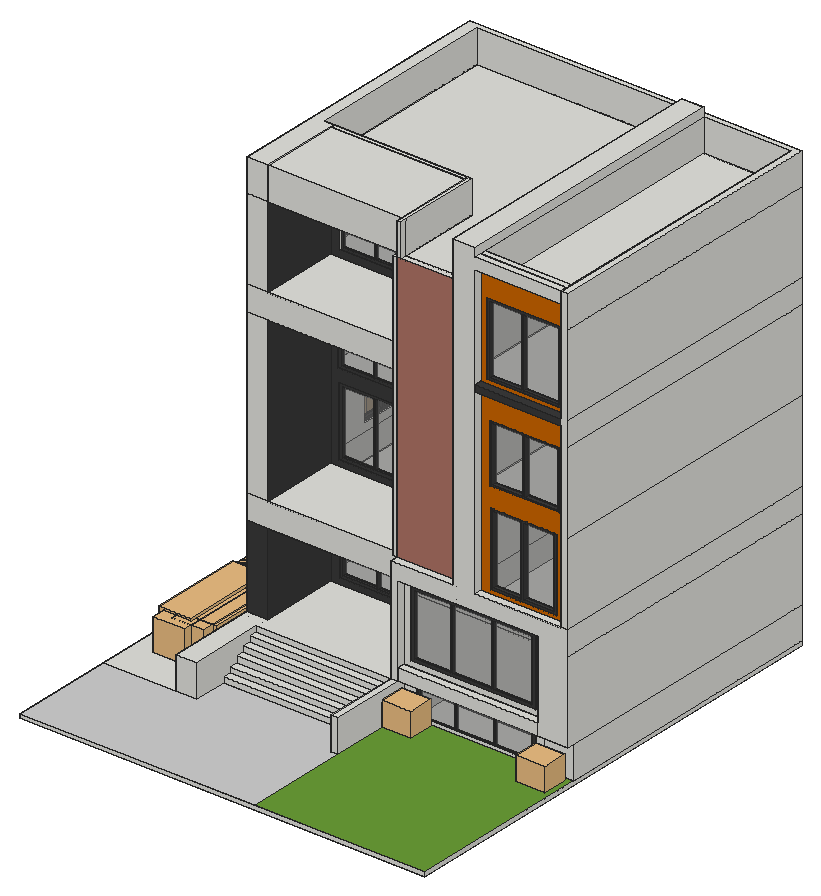
# SketchUp Ruby script. Lengths in inches.
U = 1.inch
M = Sketchup.active_model
def pt(a) = Geom::Point3d.new(a.map { |v| v * U })
def face(e, loops, mat)
  f = e.add_face(loops[0].map { |a| pt(a) })
  loops[1..].each { |l| e.add_face(l.map { |a| pt(a) }).erase! }
  f.material = f.back_material = mat if mat
  f
end
# faces: each face lists its corners as indices into pts; further lists are holes
def faces(e, pts, list, mat = nil) = list.each { |f| face(e, (f[0].is_a?(Array) ? f : [f]).map { |l| l.map { |i| pts[i] } }, mat) }
# xy, xz, yz: faces in a plane at the given z, y or x. An outline is a flat list of corners, or four numbers for a rectangle; further outlines are holes
def ring(l) = l.size == 4 ? [[l[0], l[1]], [l[2], l[1]], [l[2], l[3]], [l[0], l[3]]] : l.each_slice(2).to_a
def flat(e, list, mat, &to3) = list.each { |f| face(e, (f[0].is_a?(Array) ? f : [f]).map { |l| ring(l).map { |u, v| to3.(u, v) } }, mat) }
def xy(e, z, list, mat = nil) = flat(e, list, mat) { |x, y| [x, y, z] }
def xz(e, y, list, mat = nil) = flat(e, list, mat) { |x, z| [x, y, z] }
def yz(e, x, list, mat = nil) = flat(e, list, mat) { |y, z| [x, y, z] }
def lines(e, pts, list) = list.each { |a, b| e.add_line(pt(pts[a]), pt(pts[b])) }
# prism: a flat outline (further loops are holes) pulled along v
def prism(e, loops, v, mat = nil)
  f = face(e, loops, mat); d = Geom::Vector3d.new(v.map { |x| x * U })
  f.pushpull(f.normal.samedirection?(d) ? d.length : -d.length)
end
def box(e, o, s, mat = nil) = prism(e, [[o, [o[0] + s[0], o[1], o[2]], [o[0] + s[0], o[1] + s[1], o[2]], [o[0], o[1] + s[1], o[2]]]], [0, 0, s[2]], mat)
def at(x, y, z, deg = 0) = Geom::Transformation.translation(pt([x, y, z])) * Geom::Transformation.rotation(ORIGIN, Z_AXIS, deg.degrees)
def axes(o, x, y, z) = Geom::Transformation.new([*x, 0, *y, 0, *z, 0, *pt(o).to_a, 1])
def part(name) = M.definitions.add(name)
# library, detail: a bought-in or finely detailed component or shape, given as its bounding box
def library(name, o, s) = part(name).tap { |d| box(d.entities, o, s) }
def detail(e, o, s) = box(e.add_group.entities, o, s)
def put(e, d, t, mat = nil) = e.add_instance(d, t).tap { |i| i.material = mat if mat }
def group(e, t, mat = nil) = e.add_group.tap { |g| g.transformation = t; g.material = mat if mat }.entities
root = M.entities
M.materials.add("[Carrera Marble]").color = [207, 207, 207]
M.materials.add("[Color C06]").color = [204, 102, 0]
M.materials.add("[Color M07]").color = [58, 58, 58]
M.materials.add("[Grass Dark Green]").color = [106, 157, 55]
M.materials.add("[Groundcover Rock Crushed Multi]").color = [143, 133, 129]
M.materials.add("[Polished Concrete New]").color = [200, 200, 203]
M.materials.add("[Stone Flagstone Ashlar]").color = [175, 116, 102]
M.materials.add("[Translucent Glass Gray]").color = [128, 128, 128]
M.materials["[Translucent Glass Gray]"].alpha = 0.5
c1 = library("Vasos",[-24.5625,-15.95,-1.45],[31.57,37.11,26.14])
c2 = library("Leafy branch",[-35.17,-3.01,-3.57],[143.18,161.35,119.45])
c3 = library("Group\#55",[5.86,-0.04,-1.79],[34.39,19.68,504.85])
c4 = library("Group\#24",[28.02,-2.92,-0.02],[141.73,84.93,456.9])
c5 = library("Group\#66",[-11.6875,-1.03,-0.36],[108.82,105.43,84.06])
c6 = library("Group\#74",[28.02,-2.92,-0.02],[141.73,84.93,456.9])
c7 = library("Group\#19",[-11.6875,-1.03,-0.36],[108.82,105.43,84.06])
c8 = library("Group\#65",[-11.6875,-1.03,-0.36],[108.82,105.43,84.06])
c9 = part("BROADLEAF TREE 4")
g1 = group(c9.entities,at(835.71,714.57,-6.32))
put(g1,c2,at(175.35,181.4,81.93,-120))
put(g1,c2,at(98.01,135.17,98.79))
put(g1,c2,at(125.27,89.16,75.51,60))
put(g1,c3,axes([114.37,132.6,1.2],[1.053,0,0],[0,0.702,0],[0,0,0.67275]))
g2 = group(g1,at(131.4375,132.24,187.74))
detail(g2,[0.38,-62.11,4.18],[9.04,69.09,65.1])
g3 = group(g1,at(138.38,139.84,128.99))
detail(g3,[-52.45,-27.55,5.12],[58.39,28.31,68.09])
g4 = group(g1,at(143.59,136.18,156.43))
p = [[-4.06,0.97,6.8125],[-3.16,1.92,5.12],[16.64,3.22,19.03],[-3.46,4.03,5.3],[17.74,5.76,18.54],[18.03,4.05,18.38],
  [-4.55,4.39,7.11],[16.17,5.98,19.27],[-4.92,2.5,8.04],[15.5,4.41,19.57],[23.5,3.0625,29.43],[23.29,4.375,29.58],
  [22.46,2.41,29.96],[21.6,3.33,30.42],[22.12,4.54,30.1875],[29.5,2.95,39.79],[28.53,2.3,40.45],[29.28,4.27,39.92],
  [28.18,4.43,40.65],[27.71,3.22,40.98],[31.53,2.38,43.47],[32.65,3.05,43.15],[32.44,4.36,43.34],[31.2,4.5,43.77],
  [30.63,3.28,43.86],[33.92,2.08,46.91],[32.76,1.45,47.125],[33.71,3.39,47.09],[32.43,3.57,47.41],[31.84,2.36,47.43],
  [34.82,1.94,50.6],[33.66,1.3,50.81],[34.59,3.25,50.68],[32.72,2.22,51.03],[33.29,3.42,50.95],[36.53,1.65,58.5],
  [36.33,2.72,58.51],[35.58,1.14,58.62],[34.79,1.89,58.7],[35.26,2.86,58.64],[35.46,1.38,65.01],[35.43,2.21,71.12],
  [36.63,2.02,64.94],[36.14,2.61,70.86],[36.38,3.33,64.88],[35.0625,3.51,64.91],[34.49,2.3,64.99],[34.85,2.8,71.32],
  [35.19,3.58,71.18],[35.99,3.46,70.89],[40.53,1.63,83.61],[40.25,1.48,83.71],[40.48,1.96,83.65],[40.17,2,83.77],
  [40.03,1.7,83.81]]
faces(g4,p,[[0,1,2],[3,4,1],[5,1,4],[5,2,1],[6,7,3],[4,3,7],[0,2,8],[6,8,7],
  [9,8,2],[9,7,8],[5,10,2],[4,11,10,5],[4,7,11],[2,12,9],[12,2,10],[7,9,13,14],
  [14,11,7],[13,9,12],[12,10,15,16],[10,11,17,15],[11,14,18,17],[13,12,16,19],[14,13,19,18],[16,15,20],
  [21,20,15],[17,22,15],[21,15,22],[18,23,22,17],[19,16,24],[20,24,16],[18,19,23],[24,23,19],
  [20,21,25,26],[21,22,27,25],[22,23,28,27],[24,20,26,29],[23,24,29,28],[26,25,30,31],[25,27,32,30],[29,26,31,33],
  [27,28,34,32],[28,29,33,34],[30,35,31],[35,30,36],[32,36,30],[32,34,36],[31,37,33],[37,31,35],
  [34,33,38,39],[39,36,34],[38,33,37],[37,35,40],[40,35,41],[35,42,41],[35,36,42],[42,36,43],
  [36,44,43],[39,45,36],[44,36,45],[38,37,46],[40,46,37],[39,38,46],[46,47,39],[47,48,39],
  [45,39,48],[43,41,42],[49,43,44],[48,44,45],[49,44,48],[47,46,40],[41,47,40],[43,50,51,41],
  [50,43,52],[48,53,49],[52,49,53],[49,52,43],[51,54,41],[47,41,54],[48,47,53],[54,53,47]])
put(g1,c4,axes([125.48,145.0625,217.42],[0.00012,-0.14788,0.16558],[0.16656,0.10953,0.0977],[-0.12231,0.10348,0.09251]))
put(g1,c5,axes([243.09,175.3,91.11],[-0.32401,0.946,-0.00982],[-0.87686,-0.2964,0.3785],[0.35515,0.13125,0.92555]))
put(g1,c5,axes([263.78,129.89,165.3],[-0.32401,0.946,-0.00982],[-0.87686,-0.2964,0.3785],[0.35515,0.13125,0.92555]))
put(g1,c5,axes([54.24,237.85,216.29],[-0.4616,-0.88171,-0.09756],[0.69419,-0.4275,0.57908],[-0.55229,0.19958,0.80941]))
put(g1,c6,axes([118.85,136.48,268.97],[0.12801,0.07405,0.16558],[-0.17813,0.08948,0.0977],[-0.02846,-0.15766,0.09251]))
put(g1,c7,axes([27.82,157.38,137.2],[-0.28483,-0.8975,0.3367],[0.87996,-0.1055,0.46318],[-0.38018,0.42822,0.81981]))
put(g1,c5,at(-1.07,209.96,287.66,-90))
put(g1,c5,at(165.73,30.1,301.44,55))
put(g1,c5,at(72.15,28.01,172.33,5))
put(g1,c5,at(147.85,46.84,206.57,5))
put(g1,c8,axes([104.45,83.52,51.16],[0.66787,-0.70795,0.22971],[0.56151,0.68184,0.46883],[-0.48853,-0.18413,0.8529]))
put(g1,c5,at(110.39,-7.27,239.375,5))
put(g1,c5,at(153.13,245.69,272.42,165))
put(g1,c7,at(124.56,34.23,144.59,20))
put(g1,c8,axes([46.25,140.4,185.01],[0.66218,-0.71803,0.21438],[0.37449,0.5649,0.73529],[-0.64906,-0.40661,0.64296]))
put(g1,c5,at(179.25,63.58,322.81,55))
put(g1,c5,at(125.13,241.09,334.61,-155))
put(g1,c5,at(213.8,138.73,287.53,125))
put(g1,c7,at(40.15,67.87,155.05,-30))
c10 = library("chậu cây",[-51.89,-15.59,-1.68],[103.03,17.61,21.35])
c11 = part("Group\#4")
xy(c11.entities,0,[[0,0,112.4375,4.3125]],"[Color M07]")
xy(c11.entities,3.83,[[3.83,0,35.49,4.3125],[35.49,0,37.29,4.3125],[37.29,0,72.55,4.3125],[72.55,0,74.35,4.3125],[74.35,0,108.61,4.3125]],"[Color M07]")
xy(c11.entities,85.92,[[3.83,0,35.49,4.3125],[37.29,0,72.55,4.3125],[74.35,0,108.61,4.3125]],"[Color M07]")
xy(c11.entities,89.75,[[0,0,112.4375,4.3125]],"[Color M07]")
xz(c11.entities,0,[[[0,0,112.4375,89.75],[3.83,3.83,3.83,85.92,35.49,85.92,35.49,3.83,37.29,3.83,37.29,85.92,72.55,85.92,72.55,3.83,74.35,3.83,74.35,85.92,108.61,85.92,108.61,3.83]]],"[Color M07]")
xz(c11.entities,4.3125,[[[0,0,112.4375,89.75],[3.83,3.83,108.61,3.83,108.61,85.92,74.35,85.92,74.35,3.83,72.55,3.83,72.55,85.92,37.29,85.92,37.29,3.83,35.49,3.83,35.49,85.92,3.83,85.92]]],"[Color M07]")
xz(c11.entities,4.3125,[[3.83,3.83,35.49,85.92],[37.29,3.83,72.55,85.92],[74.35,3.83,108.61,85.92]],"[Translucent Glass Gray]")
yz(c11.entities,0,[[0,0,4.3125,89.75]],"[Color M07]")
yz(c11.entities,3.83,[[0,3.83,4.3125,85.92]],"[Color M07]")
yz(c11.entities,35.49,[[0,3.83,4.3125,85.92]],"[Color M07]")
yz(c11.entities,37.29,[[0,3.83,4.3125,85.92]],"[Color M07]")
yz(c11.entities,72.55,[[0,3.83,4.3125,85.92]],"[Color M07]")
yz(c11.entities,74.35,[[0,3.83,4.3125,85.92]],"[Color M07]")
yz(c11.entities,108.61,[[0,3.83,4.3125,85.92]],"[Color M07]")
yz(c11.entities,112.4375,[[0,0,4.3125,89.75]],"[Color M07]")
c12 = part("Group\#2")
xy(c12.entities,0,[[0,0,53.875,2.5]],"[Color M07]")
xy(c12.entities,1.79,[[1.79,0,25.11,2.5],[25.11,0,26.9375,2.5],[26.9375,0,52.08,2.5]],"[Color M07]")
xy(c12.entities,66.83,[[1.79,0,25.11,2.5],[26.9375,0,52.08,2.5]],"[Color M07]")
xy(c12.entities,68.625,[[0,0,53.875,2.5]],"[Color M07]")
xz(c12.entities,0,[[[0,0,53.875,68.625],[1.79,1.79,1.79,66.83,25.11,66.83,25.11,1.79,26.9375,1.79,26.9375,66.83,52.08,66.83,52.08,1.79]]],"[Color M07]")
xz(c12.entities,2.5,[[[0,0,53.875,68.625],[1.79,1.79,52.08,1.79,52.08,66.83,26.9375,66.83,26.9375,1.79,25.11,1.79,25.11,66.83,1.79,66.83]]],"[Color M07]")
xz(c12.entities,2.5,[[1.79,1.79,25.11,66.83],[26.9375,1.79,52.08,66.83]],"[Translucent Glass Gray]")
yz(c12.entities,0,[[0,0,2.5,68.625]],"[Color M07]")
yz(c12.entities,1.79,[[0,1.79,2.5,66.83]],"[Color M07]")
yz(c12.entities,25.11,[[0,1.79,2.5,66.83]],"[Color M07]")
yz(c12.entities,26.9375,[[0,1.79,2.5,66.83]],"[Color M07]")
yz(c12.entities,52.08,[[0,1.79,2.5,66.83]],"[Color M07]")
yz(c12.entities,53.875,[[0,0,2.5,68.625]],"[Color M07]")
c13 = part("Group\#1")
xy(c13.entities,0,[[0,0,112.4375,4.3125]],"[Color M07]")
xy(c13.entities,3.83,[[3.83,0,35.49,4.3125],[35.49,0,37.29,4.3125],[37.29,0,72.55,4.3125],[72.55,0,74.35,4.3125],[74.35,0,108.61,4.3125]],"[Color M07]")
xy(c13.entities,85.92,[[3.83,0,35.49,4.3125],[37.29,0,72.55,4.3125],[74.35,0,108.61,4.3125]],"[Color M07]")
xy(c13.entities,89.75,[[0,0,112.4375,4.3125]],"[Color M07]")
xz(c13.entities,0,[[[0,0,112.4375,89.75],[3.83,3.83,3.83,85.92,35.49,85.92,35.49,3.83,37.29,3.83,37.29,85.92,72.55,85.92,72.55,3.83,74.35,3.83,74.35,85.92,108.61,85.92,108.61,3.83]]],"[Color M07]")
xz(c13.entities,4.3125,[[[0,0,112.4375,89.75],[3.83,3.83,108.61,3.83,108.61,85.92,74.35,85.92,74.35,3.83,72.55,3.83,72.55,85.92,37.29,85.92,37.29,3.83,35.49,3.83,35.49,85.92,3.83,85.92]]],"[Color M07]")
xz(c13.entities,4.3125,[[3.83,3.83,35.49,85.92],[37.29,3.83,72.55,85.92],[74.35,3.83,108.61,85.92]],"[Translucent Glass Gray]")
yz(c13.entities,0,[[0,0,4.3125,89.75]],"[Color M07]")
yz(c13.entities,3.83,[[0,3.83,4.3125,85.92]],"[Color M07]")
yz(c13.entities,35.49,[[0,3.83,4.3125,85.92]],"[Color M07]")
yz(c13.entities,37.29,[[0,3.83,4.3125,85.92]],"[Color M07]")
yz(c13.entities,72.55,[[0,3.83,4.3125,85.92]],"[Color M07]")
yz(c13.entities,74.35,[[0,3.83,4.3125,85.92]],"[Color M07]")
yz(c13.entities,108.61,[[0,3.83,4.3125,85.92]],"[Color M07]")
yz(c13.entities,112.4375,[[0,0,4.3125,89.75]],"[Color M07]")
c14 = part("Group\#3")
xy(c14.entities,0,[[0,0,2.6875,65.5]],"[Color M07]")
xy(c14.entities,2.48,[[0,2.48,2.6875,33.53],[0,35.17,2.6875,63.02]],"[Color M07]")
xy(c14.entities,70.4,[[0,2.48,2.6875,33.53],[0,35.17,2.6875,63.02]],"[Color M07]")
xy(c14.entities,72.875,[[0,0,2.6875,65.5]],"[Color M07]")
xz(c14.entities,0,[[0,0,2.6875,72.875]],"[Color M07]")
xz(c14.entities,2.48,[[0,2.48,2.6875,70.4]],"[Color M07]")
xz(c14.entities,33.53,[[0,2.48,2.6875,70.4]],"[Color M07]")
xz(c14.entities,35.17,[[0,2.48,2.6875,70.4]],"[Color M07]")
xz(c14.entities,63.02,[[0,2.48,2.6875,70.4]],"[Color M07]")
xz(c14.entities,65.5,[[0,0,2.6875,72.875]],"[Color M07]")
yz(c14.entities,0,[[[0,0,65.5,72.875],[2.48,2.48,33.53,70.4],[35.17,2.48,63.02,70.4]]],"[Color M07]")
yz(c14.entities,0,[[2.48,2.48,33.53,70.4],[35.17,2.48,63.02,70.4]],"[Translucent Glass Gray]")
yz(c14.entities,2.6875,[[[0,0,65.5,72.875],[2.48,2.48,33.53,70.4],[35.17,2.48,63.02,70.4]]],"[Color M07]")
xy(root,0,[[124.94,0,720.75,694.9375]])
xy(root,6,[[124.94,153.1875,231.75,153.1875,231.75,228.35,158.69,228.35,158.69,648.72,231.75,648.72,231.75,694.9375,124.94,694.9375],[231.75,153.1875,231.75,381.36,240.75,381.36,240.75,274.9375,262.25,274.9375,262.25,153.1875],[460.32,153.1875,470.08,274.9375],[262.25,202.9375,460.32,214.9375],[262.25,214.9375,460.32,274.9375],
  [240.75,274.9375,240.75,564.58,231.75,564.58,231.75,694.9375,720.75,694.9375,720.75,274.9375,460.32,274.9375,460.32,275.0625,262.25,275.0625,262.25,274.9375],[262.25,274.9375,460.32,275.0625],[262.25,274.9375,460.32,275.0625],[231.75,381.36,240.75,564.58]])
xy(root,6,[[124.94,0,470.08,0,470.08,153.1875,460.32,153.1875,460.32,202.9375,262.25,202.9375,262.25,153.1875,124.94,153.1875]],"[Carrera Marble]")
xy(root,6,[[470.08,0,720.75,274.9375]],"[Grass Dark Green]")
xy(root,6,[[162.35,232,228.1,645.07]],"[Groundcover Rock Crushed Multi]")
xy(root,10.11,[[490.6,274.9375,665.78,322.6875]])
xy(root,14,[[262.25,202.9375,460.32,214.9375]])
xy(root,18,[[[158.69,228.35,231.75,648.72],[162.35,232,228.1,645.07]]],"[Polished Concrete New]")
xy(root,22,[[262.25,214.9375,460.32,226.9375]])
xy(root,30,[[262.25,226.9375,460.32,238.9375]])
xy(root,38,[[262.25,238.9375,460.32,250.9375]])
xy(root,43.4375,[[231.75,466.16,240.75,564.58]])
xy(root,46,[[262.25,250.9375,460.32,262.9375]])
xy(root,48.8,[[490.6,274.9375,665.78,322.6875]])
xy(root,54,[[231.75,153.1875,262.25,153.1875,262.25,262.9375,460.32,262.9375,460.32,399.9375,263.32,399.9375,263.32,283.9375,231.75,283.9375],[460.32,153.1875,470.08,263.6875],[460.32,263.6875,470.08,274.9375],[470.08,263.6875,720.75,274.9375],[466.32,283.9375,711.75,283.9375,711.75,685.9375,249.75,685.9375,249.75,405.9375,466.32,405.9375]])
xy(root,54,[[231.75,283.9375,240.75,381.36],[231.75,381.36,240.75,466.16]],"[Color M07]")
xy(root,62.25,[[231.75,602.51,249.75,680.81]])
xy(root,62.93,[[275.43,399.9375,448.37,405.9375]])
xy(root,64.9375,[[231.75,466.16,240.75,564.58]])
xy(root,65.25,[[231.75,602.51,249.75,680.81]])
xy(root,67.9375,[[231.75,466.16,240.75,564.58]])
xy(root,70.06,[[240.75,476.58,249.75,553.46]])
xy(root,72.0625,[[470.08,263.6875,676.93,274.9375]])
xy(root,79.55,[[480.64,274.9375,664.7,283.9375]])
xy(root,160.31,[[240.75,476.58,249.75,553.46]])
xy(root,162.75,[[466.32,283.9375,466.32,405.9375,249.75,405.9375,249.75,685.9375,711.75,685.9375,711.75,283.9375]])
xy(root,165.12,[[275.43,399.9375,448.37,405.9375]])
xy(root,168,[[466.32,283.9375,711.75,283.9375,711.75,685.9375,249.75,685.9375,249.75,405.9375,466.32,405.9375]])
xy(root,174,[[466.32,283.9375,556.88,283.9375,556.88,685.9375,249.75,685.9375,249.75,405.9375,466.32,405.9375],[556.88,283.9375,562.88,685.9375],[231.75,466.16,240.75,564.58],[231.75,602.51,249.75,680.81],[231.75,680.81,240.75,694.9375]])
xy(root,174,[[263.32,283.9375,460.32,399.9375]],"[Color M07]")
xy(root,178.93,[[480.64,274.9375,664.7,283.9375]])
xy(root,186.375,[[470.08,263.6875,676.93,274.9375]])
xy(root,193.8125,[[229.07,602.51,231.75,694.9375]],"[Color M07]")
xy(root,196.08,[[229.07,602.51,231.75,694.9375]],"[Color M07]")
xy(root,210,[[460.32,263.6875,551.32,274.9375],[583.88,263.6875,711.75,274.9375],[711.75,263.6875,720.75,274.9375],[454.07,274.9375,460.32,283.9375],[263.32,283.9375,454.07,399.9375],
  [454.07,283.9375,460.32,399.9375],[231.75,466.16,240.75,564.58],[231.75,602.51,240.75,680.81],[240.75,602.51,249.75,680.81],[231.75,680.81,240.75,694.9375]])
xy(root,213,[[231.75,466.16,240.75,564.58],[231.75,602.51,240.75,680.81]])
xy(root,215.2,[[598.53,274.9375,695.53,283.9375]])
xy(root,218.42,[[274.35,399.9375,437.54,405.9375]])
xy(root,222.99,[[240.75,476.58,249.75,553.46]])
xy(root,313.24,[[240.75,476.58,249.75,553.46]])
xy(root,320.98,[[274.35,399.9375,437.54,405.9375]])
xy(root,323.33,[[598.53,274.9375,695.53,283.9375]])
xy(root,324,[[466.32,283.9375,466.32,405.9375,249.75,405.9375,249.75,685.9375,556.88,685.9375,556.88,283.9375],[562.88,283.9375,711.75,685.9375]])
xy(root,330,[[466.32,283.9375,556.88,283.9375,556.88,685.9375,249.75,685.9375,249.75,405.9375,466.32,405.9375],[562.88,283.9375,711.75,685.9375],[231.75,466.16,240.75,564.58],[231.75,602.51,249.75,680.81],[231.75,680.81,240.75,694.9375]])
xy(root,339.43,[[273.23,399.9375,437.54,405.9375]])
xy(root,346.8125,[[228.5,602.51,231.75,694.9375]],"[Color M07]")
xy(root,349.08,[[228.5,602.51,231.75,694.9375]],"[Color M07]")
xy(root,352.28,[[596.96,274.9375,700.9,283.9375]])
xy(root,361.16,[[231.75,466.16,240.75,564.58],[231.75,602.51,240.75,680.37],[240.75,602.51,249.75,680.37]])
xy(root,364.16,[[231.75,466.16,240.75,564.58],[231.75,602.51,240.75,680.37]])
xy(root,371.86,[[240.75,483.68,249.75,548.93]])
xy(root,437.11,[[240.75,483.68,249.75,548.93]])
xy(root,437.43,[[273.23,399.9375,437.54,405.9375]])
xy(root,438.78,[[596.96,274.9375,700.9,283.9375]])
xy(root,450,[[454.07,283.9375,460.32,399.9375],[231.75,466.16,240.75,564.58],[231.75,602.51,249.75,680.37]])
xy(root,450,[[263.32,283.9375,454.07,399.9375]],"[Color M07]")
xy(root,473.3125,[[562.88,283.9375,711.75,685.9375]])
xy(root,475.68,[[583.88,263.6875,711.75,274.9375]],"[Color M07]")
xy(root,480,[[466.32,283.9375,466.32,405.9375,249.75,405.9375,249.75,685.9375,556.88,685.9375,556.88,283.9375]])
xy(root,486,[[466.32,283.9375,556.88,283.9375,556.88,685.9375,249.75,685.9375,249.75,405.9375,466.32,405.9375],[263.32,283.9375,454.07,399.9375],[454.07,283.9375,460.32,399.9375],[562.88,283.9375,711.75,685.9375],[231.75,466.16,240.75,564.58],
  [231.75,602.51,249.75,680.81]])
xy(root,486,[[583.88,263.6875,711.75,274.9375]],"[Color M07]")
xy(root,489,[[231.75,466.16,240.75,564.58],[231.75,602.51,249.75,680.81]])
xy(root,492.22,[[593.2,274.9375,702.08,283.9375]])
xy(root,495.92,[[276.53,399.9375,437.54,405.9375]])
xy(root,499.12,[[240.75,476.58,249.75,553.46]])
xy(root,589.37,[[240.75,476.58,249.75,553.46]])
xy(root,596.04,[[276.53,399.9375,437.54,405.9375]])
xy(root,598.28,[[593.2,274.9375,702.08,283.9375]])
xy(root,600,[[466.32,283.9375,466.32,405.9375,249.75,405.9375,249.75,685.9375,556.88,685.9375,556.88,283.9375],[562.88,283.9375,711.75,685.9375]])
xy(root,606,[[454.07,274.9375,460.32,283.9375],[460.32,274.9375,466.32,405.9375],[466.32,274.9375,551.32,283.9375],[551.32,274.9375,556.88,283.9375],[466.32,283.9375,551.32,283.9375,551.32,685.9375,249.75,685.9375,249.75,405.9375,466.32,405.9375],
  [454.07,283.9375,460.32,399.9375],[551.32,283.9375,556.88,685.9375],[562.88,283.9375,583.88,685.9375],[583.88,283.9375,711.75,685.9375],[263.32,399.9375,460.32,405.9375],
  [231.75,466.16,240.75,564.58],[231.75,602.51,249.75,680.81]])
xy(root,606,[[263.32,283.9375,454.07,399.9375]],"[Color M07]")
xy(root,636.96,[[583.88,263.6875,711.75,274.9375]])
xy(root,654,[[711.75,263.6875,720.75,263.6875,720.75,694.9375,231.75,694.9375,231.75,283.9375,263.32,283.9375,263.32,405.9375,249.75,405.9375,249.75,685.9375,711.75,685.9375],[583.88,263.6875,711.75,274.9375],[460.32,274.9375,466.32,405.9375],[556.88,274.9375,562.88,274.9375,562.88,283.9375,583.88,283.9375,583.88,685.9375,556.88,685.9375],[562.88,274.9375,583.88,283.9375],
  [583.88,274.9375,711.75,283.9375],[263.32,283.9375,460.32,399.9375],[263.32,399.9375,460.32,405.9375]])
xy(root,667,[[551.32,263.6875,583.88,685.9375]])
xz(root,0,[[124.94,0,720.75,6]])
xz(root,153.1875,[[231.75,6,262.25,54],[460.32,6,470.08,54]])
xz(root,202.9375,[[262.25,6,460.32,14]])
xz(root,214.9375,[[262.25,14,460.32,22]])
xz(root,226.9375,[[262.25,22,460.32,30]])
xz(root,228.35,[[158.69,6,231.75,18]],"[Polished Concrete New]")
xz(root,232,[[162.35,6,228.1,18]],"[Polished Concrete New]")
xz(root,238.9375,[[262.25,30,460.32,38]])
xz(root,250.9375,[[262.25,38,460.32,46]])
xz(root,262.9375,[[262.25,46,460.32,54]])
xz(root,263.6875,[[460.32,54,470.08,54,470.08,186.375,676.93,186.375,676.93,54,720.75,54,720.75,210,583.88,210,583.88,636.96,711.75,636.96,711.75,654,583.88,654,583.88,667,551.32,667,551.32,210,460.32,210],[470.08,54,676.93,72.0625],[711.75,210,720.75,654]])
xz(root,263.6875,[[583.88,475.68,711.75,486]],"[Color M07]")
xz(root,274.9375,[[262.25,6,460.32,46],[460.32,6,470.08,54],[[470.08,6,676.93,54],[490.6,10.11,665.78,48.8]],[676.93,6,720.75,54],[470.08,54,676.93,72.0625],
  [[470.08,72.0625,676.93,186.375],[480.64,79.55,664.7,178.93]],[454.07,210,460.32,606],[551.32,210,556.88,330],[551.32,330,556.88,450],[551.32,450,556.88,486],
  [551.32,486,556.88,606],[460.32,606,466.32,654],[556.88,606,562.88,654],[562.88,606,583.88,606,583.88,636.96,711.75,636.96,711.75,654,562.88,654]])
xz(root,274.9375,[[[583.88,210,711.75,475.68],[598.53,215.2,695.53,323.33],[596.96,352.28,700.9,438.78]],[[583.88,486,711.75,636.96],[593.2,492.22,702.08,598.28]]],"[Color C06]")
xz(root,274.9375,[[460.32,210,551.32,606]],"[Stone Flagstone Ashlar]")
xz(root,283.9375,[[466.32,54,466.32,162.75,480.64,162.75,480.64,79.55,664.7,79.55,664.7,162.75,711.75,162.75,711.75,54],[480.64,79.55,664.7,162.75],[466.32,162.75,480.64,168],[480.64,162.75,664.7,168],[664.7,162.75,711.75,168],
  [466.32,168,480.64,174],[480.64,168,664.7,168,664.7,178.93,562.88,178.93,562.88,174,480.64,174],[664.7,168,664.7,178.93,562.88,178.93,562.88,210,711.75,210,711.75,168],[231.75,174,460.32,210],[466.32,174,466.32,210,556.88,210,556.88,178.93,480.64,178.93,480.64,174],
  [480.64,174,556.88,178.93],[556.88,174,562.88,178.93],[231.75,210,263.32,450],[466.32,210,556.88,324],[[562.88,210,711.75,324],[598.53,215.2,695.53,323.33]],
  [466.32,324,556.88,330],[562.88,324,711.75,330],[466.32,330,556.88,450],[[562.88,330,711.75,450],[596.96,352.28,700.9,438.78]],[231.75,450,454.07,486],
  [454.07,450,460.32,486],[466.32,450,556.88,480],[562.88,450,711.75,473.3125],[562.88,473.3125,711.75,486],[466.32,480,556.88,486],
  [231.75,486,263.32,606],[466.32,486,556.88,600],[[562.88,486,711.75,600],[593.2,492.22,702.08,598.28]],[466.32,600,556.88,606],[562.88,600,711.75,606],
  [231.75,606,263.32,654],[263.32,606,460.32,654],[583.88,606,711.75,654]])
xz(root,283.9375,[[231.75,54,263.32,174]],"[Color M07]")
xz(root,322.6875,[[490.6,10.11,665.78,48.8]])
xz(root,381.36,[[231.75,6,240.75,54]])
xz(root,399.9375,[[454.07,210,460.32,330],[454.07,330,460.32,450],[454.07,486,460.32,606],[263.32,606,460.32,654]])
xz(root,399.9375,[[[263.32,54,460.32,174],[275.43,62.93,448.37,165.12]],[[263.32,210,454.07,450],[274.35,218.42,437.54,320.98],[273.23,339.43,437.54,437.43]],[[263.32,486,454.07,606],[276.53,495.92,437.54,596.04]]],"[Color M07]")
xz(root,405.9375,[[249.75,54,249.75,162.75,275.43,162.75,275.43,62.93,448.37,62.93,448.37,162.75,466.32,162.75,466.32,54],[249.75,162.75,249.75,168,466.32,168,466.32,162.75,448.37,162.75,448.37,165.12,275.43,165.12,275.43,162.75],[275.43,162.75,448.37,165.12],[249.75,168,466.32,174],[249.75,174,466.32,210],
  [[249.75,210,466.32,324],[274.35,218.42,437.54,320.98]],[249.75,324,466.32,330],[[249.75,330,466.32,450],[273.23,339.43,437.54,437.43]],[249.75,450,466.32,480],[249.75,480,466.32,486],
  [[249.75,486,466.32,600],[276.53,495.92,437.54,596.04]],[249.75,600,466.32,606],[249.75,606,263.32,654],[263.32,606,460.32,654],[460.32,606,466.32,654]])
xz(root,466.16,[[231.75,43.4375,240.75,54],[231.75,54,240.75,64.9375],[231.75,64.9375,240.75,67.9375],[231.75,67.9375,240.75,174],[231.75,174,240.75,210],
  [231.75,210,240.75,213],[231.75,213,240.75,330],[231.75,330,240.75,361.16],[231.75,361.16,240.75,364.16],[231.75,364.16,240.75,450],
  [231.75,450,240.75,486],[231.75,486,240.75,489],[231.75,489,240.75,606]])
xz(root,476.58,[[240.75,70.06,249.75,160.31],[240.75,222.99,249.75,313.24],[240.75,499.12,249.75,589.37]])
xz(root,483.68,[[240.75,371.86,249.75,437.11]])
xz(root,548.93,[[240.75,371.86,249.75,437.11]])
xz(root,553.46,[[240.75,70.06,249.75,160.31],[240.75,222.99,249.75,313.24],[240.75,499.12,249.75,589.37]])
xz(root,564.58,[[231.75,43.4375,240.75,64.9375],[231.75,64.9375,240.75,67.9375],[231.75,67.9375,240.75,174],[231.75,174,240.75,210],[231.75,210,240.75,213],
  [231.75,213,240.75,330],[231.75,330,240.75,361.16],[231.75,361.16,240.75,364.16],[231.75,450,240.75,486],[231.75,486,240.75,489]])
xz(root,564.58,[[231.75,6,240.75,43.4375],[231.75,364.16,240.75,450],[231.75,489,240.75,606]],"[Color M07]")
xz(root,602.51,[[231.75,6,240.75,62.25],[231.75,62.25,240.75,65.25],[240.75,62.25,249.75,65.25],[231.75,174,240.75,210],[231.75,210,240.75,213],
  [231.75,330,240.75,361.16],[231.75,361.16,240.75,364.16],[231.75,486,249.75,489]])
xz(root,602.51,[[231.75,65.25,249.75,174],[229.07,193.8125,231.75,196.08],[240.75,210,240.75,213,231.75,213,231.75,330,249.75,330,249.75,210],[228.5,346.8125,231.75,349.08],[240.75,361.16,240.75,364.16,231.75,364.16,231.75,450,249.75,450,249.75,361.16],
  [231.75,489,249.75,606]],"[Color M07]")
xz(root,645.07,[[162.35,6,228.1,18]],"[Polished Concrete New]")
xz(root,648.72,[[158.69,6,231.75,18]],"[Polished Concrete New]")
xz(root,680.37,[[231.75,361.16,240.75,364.16],[240.75,361.16,249.75,361.16,249.75,450,231.75,450,231.75,364.16,240.75,364.16]])
xz(root,680.81,[[231.75,62.25,240.75,65.25],[240.75,62.25,249.75,65.25],[231.75,65.25,249.75,174],[231.75,210,240.75,213],[240.75,210,249.75,210,249.75,330,231.75,330,231.75,213,240.75,213],
  [231.75,486,249.75,489],[231.75,489,249.75,600],[231.75,600,249.75,606]])
xz(root,685.9375,[[249.75,54,711.75,162.75],[249.75,162.75,302.82,168],[302.82,162.75,711.75,168],[249.75,168,302.82,174],[302.82,168,711.75,174],
  [249.75,174,556.88,210],[562.88,174,711.75,210],[249.75,210,556.88,324],[562.88,210,711.75,324],[249.75,324,373.63,330],
  [373.63,324,394.19,330],[394.19,324,556.88,330],[562.88,324,573.66,330],[573.66,324,600.16,330],[600.16,324,711.75,330],
  [249.75,330,556.88,450],[562.88,330,711.75,450],[249.75,450,556.88,480],[562.88,450,711.75,473.3125],[562.88,473.3125,651.65,486],
  [651.65,473.3125,684.71,486],[684.71,473.3125,711.75,486],[249.75,480,336.08,486],[336.08,480,360.89,486],[360.89,480,556.88,486],
  [249.75,486,556.88,600],[562.88,486,711.75,600],[249.75,600,305.62,606],[305.62,600,352.24,606],[352.24,600,556.88,606],
  [562.88,600,585.84,606],[585.84,600,599.9,606],[599.9,600,711.75,606],[249.75,606,551.32,654],[551.32,606,556.88,654],
  [583.88,606,711.75,654],[551.32,654,583.88,667]])
xz(root,694.9375,[[124.94,0,720.75,6],[231.75,6,720.75,54],[231.75,54,720.75,174],[231.75,174,720.75,210],[231.75,210,720.75,330],
  [231.75,330,720.75,450],[231.75,450,720.75,486],[231.75,486,720.75,606],[231.75,606,720.75,654]])
xz(root,694.9375,[[229.07,193.8125,231.75,196.08],[228.5,346.8125,231.75,349.08]],"[Color M07]")
yz(root,124.94,[[0,0,694.9375,6]])
yz(root,158.69,[[228.35,6,648.72,18]],"[Polished Concrete New]")
yz(root,162.35,[[232,6,645.07,18]],"[Polished Concrete New]")
yz(root,228.1,[[232,6,645.07,18]],"[Polished Concrete New]")
yz(root,228.5,[[602.51,346.8125,694.9375,349.08]],"[Color M07]")
yz(root,229.07,[[602.51,193.8125,694.9375,196.08]],"[Color M07]")
yz(root,231.75,[[153.1875,6,153.1875,54,381.36,54,381.36,18,228.35,18,228.35,6],[648.72,6,648.72,18,602.51,18,602.51,62.25,694.9375,62.25,694.9375,6],[466.16,43.4375,564.58,64.9375],[602.51,62.25,680.81,65.25],[680.81,62.25,694.9375,174],
  [466.16,64.9375,564.58,67.9375],[283.9375,174,466.16,210],[466.16,174,564.58,210],[602.51,174,694.9375,193.8125],[602.51,196.08,694.9375,210],
  [466.16,210,564.58,213],[602.51,210,680.81,213],[680.81,210,694.9375,330],[466.16,330,564.58,361.16],[602.51,330,694.9375,346.8125],
  [602.51,349.08,694.9375,361.16],[466.16,361.16,564.58,364.16],[602.51,361.16,680.37,364.16],[680.37,361.16,694.9375,450],[283.9375,450,466.16,486],
  [466.16,450,564.58,486],[602.51,450,694.9375,486],[466.16,486,564.58,489],[602.51,486,680.81,489],[680.81,486,694.9375,606],
  [466.16,606,564.58,654],[602.51,606,694.9375,654]])
yz(root,231.75,[[381.36,18,381.36,54,466.16,54,466.16,43.4375,564.58,43.4375,564.58,18],[564.58,18,602.51,654],[283.9375,54,466.16,174],[602.51,193.8125,694.9375,196.08],[283.9375,210,466.16,450],
  [602.51,346.8125,694.9375,349.08],[283.9375,486,466.16,654]],"[Color M07]")
yz(root,231.75,[[228.35,6,381.36,18],[381.36,6,564.58,18],[564.58,6,602.51,18],[602.51,6,648.72,18]],"[Polished Concrete New]")
yz(root,240.75,[[466.16,43.4375,564.58,64.9375],[466.16,64.9375,564.58,67.9375],[[466.16,67.9375,564.58,174],[476.58,70.06,553.46,160.31]],[466.16,174,564.58,210],[466.16,210,564.58,213],
  [602.51,210,680.81,213],[[466.16,213,564.58,330],[476.58,222.99,553.46,313.24]],[466.16,330,564.58,361.16],[466.16,361.16,564.58,364.16],[602.51,361.16,680.37,364.16],
  [[466.16,364.16,564.58,450],[483.68,371.86,548.93,437.11]],[466.16,450,564.58,486],[466.16,486,564.58,489],[[466.16,489,564.58,606],[476.58,499.12,553.46,589.37]]])
yz(root,240.75,[[381.36,6,381.36,54,466.16,54,466.16,43.4375,564.58,43.4375,564.58,6]],"[Color M07]")
yz(root,249.75,[[[405.9375,54,685.9375,54,685.9375,162.75,680.81,162.75,680.81,62.25,602.51,62.25,602.51,162.75,405.9375,162.75],[476.58,70.06,553.46,160.31]],[602.51,62.25,680.81,65.25],[602.51,65.25,680.81,162.75],[405.9375,162.75,602.51,168],[602.51,162.75,680.81,168],
  [680.81,162.75,685.9375,168],[405.9375,168,602.51,174],[602.51,168,680.81,174],[680.81,168,685.9375,174],[405.9375,174,685.9375,210],
  [[405.9375,210,602.51,324],[476.58,222.99,553.46,313.24]],[602.51,210,680.81,324],[680.81,210,685.9375,324],[405.9375,324,602.51,330],[602.51,324,680.81,330],
  [680.81,324,685.9375,330],[[405.9375,330,685.9375,330,685.9375,450,680.37,450,680.37,361.16,602.51,361.16,602.51,450,405.9375,450],[483.68,371.86,548.93,437.11]],[405.9375,450,685.9375,480],[405.9375,480,685.9375,486],[[405.9375,486,602.51,600],[476.58,499.12,553.46,589.37]],
  [602.51,486,680.81,489],[680.81,486,685.9375,600],[602.51,489,680.81,600],[405.9375,600,602.51,606],[602.51,600,680.81,606],
  [680.81,600,685.9375,606],[405.9375,606,685.9375,654]])
yz(root,262.25,[[153.1875,6,202.9375,6,202.9375,14,214.9375,14,214.9375,22,226.9375,22,226.9375,30,238.9375,30,238.9375,38,250.9375,38,250.9375,46,262.9375,46,262.9375,54,153.1875,54],[274.9375,6,274.9375,46,275.0625,6]])
yz(root,263.32,[[283.9375,606,399.9375,654],[399.9375,606,405.9375,654]])
yz(root,263.32,[[283.9375,54,399.9375,174],[283.9375,210,399.9375,450],[283.9375,486,399.9375,606]],"[Color M07]")
yz(root,273.23,[[399.9375,339.43,405.9375,437.43]])
yz(root,274.35,[[399.9375,218.42,405.9375,320.98]])
yz(root,275.43,[[399.9375,62.93,405.9375,165.12]])
yz(root,276.53,[[399.9375,495.92,405.9375,596.04]])
yz(root,437.54,[[399.9375,218.42,405.9375,320.98],[399.9375,339.43,405.9375,437.43],[399.9375,495.92,405.9375,596.04]])
yz(root,448.37,[[399.9375,62.93,405.9375,165.12]])
yz(root,454.07,[[274.9375,210,274.9375,606,399.9375,606,399.9375,486,283.9375,486,283.9375,450,399.9375,450,399.9375,210]],"[Stone Flagstone Ashlar]")
yz(root,460.32,[[153.1875,6,153.1875,54,262.9375,54,262.9375,46,250.9375,46,250.9375,38,238.9375,38,238.9375,30,226.9375,30,226.9375,22,214.9375,22,214.9375,14,202.9375,14,202.9375,6],[202.9375,6,202.9375,14,214.9375,14,214.9375,22,226.9375,22,226.9375,30,238.9375,30,238.9375,38,250.9375,38,250.9375,46,262.9375,46,262.9375,54,274.9375,54,274.9375,6],[274.9375,6,275.0625,6,274.9375,46],[263.6875,54,263.6875,210,283.9375,210,283.9375,174,337.4375,174,337.4375,54],[274.9375,210,399.9375,210,399.9375,450,283.9375,450,283.9375,486,399.9375,486,399.9375,606,274.9375,606],
  [274.9375,606,283.9375,654],[283.9375,606,399.9375,654],[399.9375,606,405.9375,654]])
yz(root,460.32,[[337.4375,54,399.9375,174]],"[Stone Flagstone Ashlar]")
yz(root,466.32,[[283.9375,54,405.9375,162.75],[283.9375,162.75,405.9375,168],[283.9375,168,405.9375,174],[283.9375,174,405.9375,210],[283.9375,210,405.9375,324],
  [283.9375,324,405.9375,330],[283.9375,330,405.9375,450],[283.9375,450,405.9375,480],[283.9375,480,405.9375,486],[283.9375,486,405.9375,600],
  [283.9375,600,405.9375,606],[274.9375,606,283.9375,654],[283.9375,606,405.9375,654]])
yz(root,470.08,[[153.1875,6,274.9375,54],[263.6875,54,274.9375,72.0625],[263.6875,72.0625,274.9375,186.375]])
yz(root,480.64,[[274.9375,79.55,283.9375,178.93]])
yz(root,490.6,[[274.9375,10.11,322.6875,48.8]])
yz(root,551.32,[[263.6875,513.68,263.6875,667,685.9375,667,685.9375,606,274.9375,606,274.9375,513.68]])
yz(root,551.32,[[263.6875,210,274.9375,513.68]],"[Stone Flagstone Ashlar]")
yz(root,556.88,[[283.9375,174,685.9375,210],[274.9375,210,283.9375,606],[283.9375,210,685.9375,324],[283.9375,324,685.9375,330],[283.9375,330,685.9375,450],
  [283.9375,450,685.9375,480],[283.9375,480,685.9375,486],[283.9375,486,685.9375,600],[283.9375,600,685.9375,606],[274.9375,606,283.9375,654],
  [283.9375,606,685.9375,654]])
yz(root,562.88,[[283.9375,174,685.9375,210],[283.9375,210,685.9375,324],[283.9375,324,685.9375,330],[283.9375,330,685.9375,450],[283.9375,450,685.9375,473.3125],
  [283.9375,473.3125,685.9375,486],[283.9375,486,685.9375,600],[283.9375,600,685.9375,606]])
yz(root,583.88,[[263.6875,210,274.9375,475.68],[263.6875,475.68,274.9375,486],[263.6875,486,274.9375,636.96],[283.9375,606,685.9375,654],[263.6875,654,685.9375,667]])
yz(root,593.2,[[274.9375,492.22,283.9375,598.28]])
yz(root,596.96,[[274.9375,352.28,283.9375,438.78]])
yz(root,598.53,[[274.9375,215.2,283.9375,323.33]])
yz(root,664.7,[[274.9375,79.55,283.9375,178.93]])
yz(root,665.78,[[274.9375,10.11,322.6875,48.8]])
yz(root,676.93,[[263.6875,72.0625,274.9375,186.375]])
yz(root,695.53,[[274.9375,215.2,283.9375,323.33]])
yz(root,700.9,[[274.9375,352.28,283.9375,438.78]])
yz(root,702.08,[[274.9375,492.22,283.9375,598.28]])
yz(root,711.75,[[283.9375,54,685.9375,162.75],[283.9375,162.75,685.9375,168],[283.9375,168,685.9375,174],[283.9375,174,685.9375,210],[263.6875,210,274.9375,475.68],
  [283.9375,210,685.9375,324],[283.9375,324,685.9375,330],[283.9375,330,685.9375,450],[283.9375,450,685.9375,473.3125],[283.9375,473.3125,685.9375,486],
  [263.6875,486,274.9375,636.96],[283.9375,486,685.9375,600],[283.9375,600,685.9375,606],[274.9375,606,283.9375,654],[283.9375,606,685.9375,654],
  [263.6875,636.96,274.9375,654]])
yz(root,720.75,[[0,0,694.9375,6],[274.9375,6,694.9375,54],[263.6875,54,694.9375,174],[263.6875,174,694.9375,210],[263.6875,210,694.9375,330],
  [263.6875,330,694.9375,450],[263.6875,450,694.9375,486],[263.6875,486,694.9375,606],[263.6875,606,694.9375,654]])
p = [[460.32,274.9375,46],[460.32,275.0625,6],[262.25,275.0625,6],[262.25,274.9375,46],[240.75,274.9375,6],[240.75,274.9375,54],
  [556.88,274.9375,210],[556.88,274.9375,192],[676.57,274.9375,192],[676.93,274.9375,192],[556.88,263.6875,210],[556.88,263.6875,192],
  [551.32,274.9375,192],[551.32,274.9375,186.375],[240.75,694.9375,361.16],[240.75,680.37,361.16],[240.75,694.9375,62.25],[240.75,680.81,62.25],
  [262.25,274.9375,54]]
faces(root,p,[[0,1,2,3]])
lines(root,p,[[4,5],[6,7],[8,9],[6,10],[7,11],[7,12],[12,13],[14,15],[16,17],[3,18]])
put(root,c1,axes([702.67,248.46,6.52],[1.3392,0,0],[0,1,0],[0,0,1.36]))
put(root,c1,axes([502.98,251.1,7.97],[1.3392,0,0],[0,1,0],[0,0,1.36]))
put(root,c9,at(-842.09,-192.25,10.25))
put(root,c10,axes([222.7,581.34,9.68],[0,-1.32,0],[2.67,0,0],[0,0,2.19]))
put(root,c10,axes([219.08,554.97,9.68],[0,-1.32,0],[2.67,0,0],[0,0,2.19]))
put(root,c10,axes([222.7,427.06,9.68],[0,-1.32,0],[2.67,0,0],[0,0,2.19]))
put(root,c10,axes([222.7,396.81,9.68],[0,-1.32,0],[2.67,0,0],[0,0,2.19]))
put(root,c10,axes([220.67,304,9.68],[0,-1.32,0],[2.67,0,0],[0,0,2.19]))
put(root,c10,axes([214.47,287.43,9.68],[0,-1.32,0],[2.67,0,0],[0,0,2.19]))
put(root,c10,axes([200.79,578.18,3.29],[0,-1.32,0],[2.67,0,0],[0,0,2.19]))
put(root,c10,axes([193.74,556.76,3.8],[0,-1.32,0],[2.67,0,0],[0,0,2.19]))
put(root,c10,axes([193.74,530.88,3.8],[0,-1.32,0],[2.67,0,0],[0,0,2.19]))
put(root,c10,axes([191.48,416.41,9.68],[0,-1.32,0],[2.67,0,0],[0,0,2.19]))
put(root,c10,axes([191.48,394.79,9.68],[0,-1.32,0],[2.67,0,0],[0,0,2.19]))
put(root,c10,axes([188.7,295.86,12.38],[0,-1.32,0],[2.67,0,0],[0,0,2.19]))
put(root,c10,axes([195.41,275.76,9.68],[0,-1.32,0],[2.67,0,0],[0,0,2.19]))
put(root,c11,axes([275.43,399.9375,62.93],[1.53808,0,0],[0,1,0],[0,0,1.13858]))
put(root,c11,axes([274.35,400.46,218.42],[1.45136,0,0],[0,0.88,0],[0,0,1.14276]))
put(root,c11,axes([273.23,400.8,339.43],[1.46137,0,0],[0,0.8008,0],[0,0,1.09192]))
put(root,c11,axes([275.21,401.18,495.92],[1.44369,0,0],[0,0.71271,0],[0,0,1.1156]))
put(root,c12,axes([598.53,274.9375,215.29],[1.80046,0,0],[0,2.9,0],[0,0,1.5743]))
put(root,c12,axes([596.96,274.9375,352.28],[1.92923,0,0],[0,2.69584,0],[0,0,1.26047]))
put(root,c12,axes([593.2,274.9375,492.22],[2.02088,0,0],[0,2.349,0],[0,0,1.54424]))
put(root,c13,axes([480.64,275.46,79.55],[1.63702,0,0],[0,0.88,0],[0,0,1.10724]))
put(root,c14,axes([240.75,476.58,70.06],[2.19,0,0],[0,1.17366,0],[0,0,1.23842]))
put(root,c14,axes([240.75,476.58,222.99],[2.19,0,0],[0,1.17366,0],[0,0,1.23842]))
put(root,c14,axes([240.75,476.58,499.12],[2.19,0,0],[0,1.17366,0],[0,0,1.23842]))
put(root,c14,axes([241.69,484.36,371.86],[1.49008,0,0],[0,0.98588,0],[0,0,0.89537]))
put(root,c14,axes([231.75,603.93,65.25],[2.19,0,0],[0,1.17366,0],[0,0,1.49222]))
put(root,c14,axes([231.75,602.51,213],[2.19,0,0],[0,1.19539,0],[0,0,1.60549]))
put(root,c14,axes([231.75,602.51,364.16],[1.533,0,0],[0,1.18869,0],[0,0,1.17788]))
put(root,c14,axes([231.75,602.51,489],[1.533,0,0],[0,1.18869,0],[0,0,1.60549]))
put(root,c13,axes([489.84,275.22,10.11],[1.56479,0,0],[0,0.32138,0],[0,0,0.43106]))
